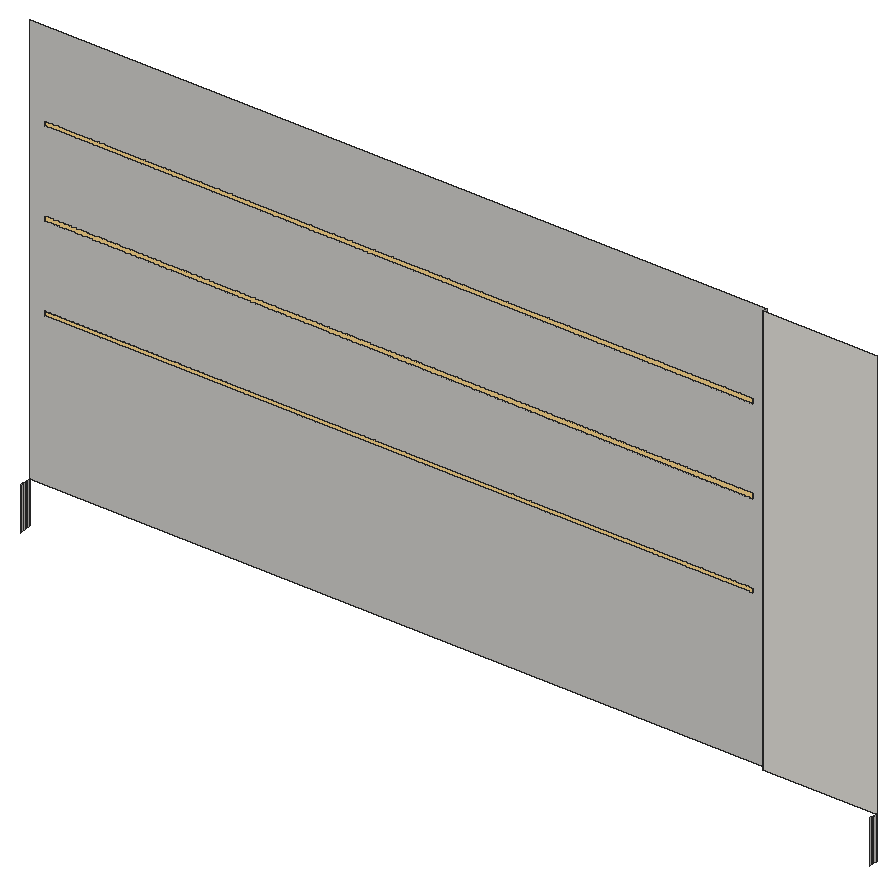
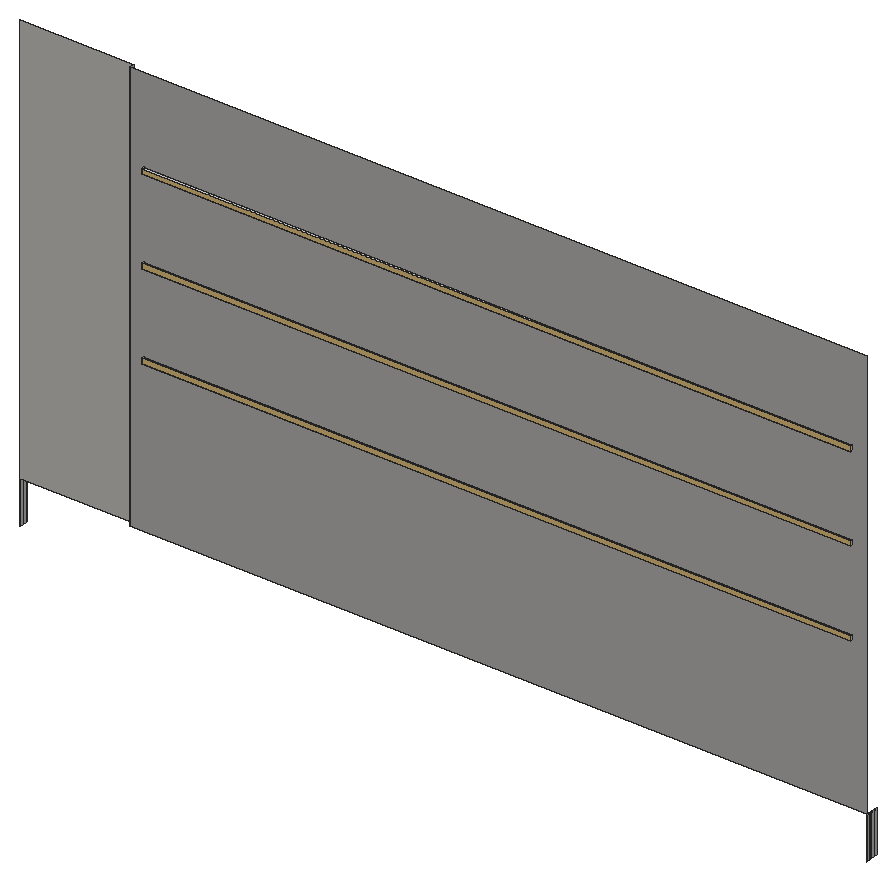
# SketchUp Ruby script. Lengths in inches.
U = 1.inch
M = Sketchup.active_model
def pt(a) = Geom::Point3d.new(a.map { |v| v * U })
def face(e, loops, mat)
  f = e.add_face(loops[0].map { |a| pt(a) })
  loops[1..].each { |l| e.add_face(l.map { |a| pt(a) }).erase! }
  f.material = f.back_material = mat if mat
  f
end
# faces: each face lists its corners as indices into pts; further lists are holes
def faces(e, pts, list, mat = nil) = list.each { |f| face(e, (f[0].is_a?(Array) ? f : [f]).map { |l| l.map { |i| pts[i] } }, mat) }
# xy, xz, yz: faces in a plane at the given z, y or x. An outline is a flat list of corners, or four numbers for a rectangle; further outlines are holes
def ring(l) = l.size == 4 ? [[l[0], l[1]], [l[2], l[1]], [l[2], l[3]], [l[0], l[3]]] : l.each_slice(2).to_a
def flat(e, list, mat, &to3) = list.each { |f| face(e, (f[0].is_a?(Array) ? f : [f]).map { |l| ring(l).map { |u, v| to3.(u, v) } }, mat) }
def xy(e, z, list, mat = nil) = flat(e, list, mat) { |x, y| [x, y, z] }
def xz(e, y, list, mat = nil) = flat(e, list, mat) { |x, z| [x, y, z] }
def yz(e, x, list, mat = nil) = flat(e, list, mat) { |y, z| [x, y, z] }
def lines(e, pts, list) = list.each { |a, b| e.add_line(pt(pts[a]), pt(pts[b])) }
# prism: a flat outline (further loops are holes) pulled along v
def prism(e, loops, v, mat = nil)
  f = face(e, loops, mat); d = Geom::Vector3d.new(v.map { |x| x * U })
  f.pushpull(f.normal.samedirection?(d) ? d.length : -d.length)
end
def box(e, o, s, mat = nil) = prism(e, [[o, [o[0] + s[0], o[1], o[2]], [o[0] + s[0], o[1] + s[1], o[2]], [o[0], o[1] + s[1], o[2]]]], [0, 0, s[2]], mat)
def at(x, y, z, deg = 0) = Geom::Transformation.translation(pt([x, y, z])) * Geom::Transformation.rotation(ORIGIN, Z_AXIS, deg.degrees)
def axes(o, x, y, z) = Geom::Transformation.new([*x, 0, *y, 0, *z, 0, *pt(o).to_a, 1])
def part(name) = M.definitions.add(name)
# library, detail: a bought-in or finely detailed component or shape, given as its bounding box
def library(name, o, s) = part(name).tap { |d| box(d.entities, o, s) }
def detail(e, o, s) = box(e.add_group.entities, o, s)
def put(e, d, t, mat = nil) = e.add_instance(d, t).tap { |i| i.material = mat if mat }
def group(e, t, mat = nil) = e.add_group.tap { |g| g.transformation = t; g.material = mat if mat }.entities
root = M.entities
M.materials.add("Outer Light - 1").color = [251, 216, 141]
M.materials.add("[Quartz Light Brown]").color = [215, 212, 212]
M.materials.add("[Stone Sandstone Ashlar Light]").color = [201, 199, 196]
M.materials.add("[Terrazzo Tile Light]").color = [219, 217, 210]
c1 = part("Group\#57")
box(c1.entities,[0,-0.5,0],[150,0.5,1])
xy(root,29,[[219,37,369,37.5]],"[Quartz Light Brown]")
xy(root,30,[[219,37,369,37.5]],"[Quartz Light Brown]")
xy(root,47,[[219,37,369,37.5]],"[Quartz Light Brown]")
xy(root,48,[[219,37,369,37.5]],"[Quartz Light Brown]")
xy(root,65,[[219,37,369,37.5]],"[Quartz Light Brown]")
xy(root,66,[[219,37,369,37.5]],"[Quartz Light Brown]")
xz(root,36,[[395.99,-12,396,-12,396,84,372,84,372,-3,395.99,-3]],"[Terrazzo Tile Light]")
xz(root,37,[[[216,-3,372,84],[219,65,369,66],[219,47,369,48],[219,29,369,30]]],"[Stone Sandstone Ashlar Light]")
xz(root,37.5,[[219,29,369,30],[219,47,369,48],[219,65,369,66]],"[Quartz Light Brown]")
yz(root,216,[[36.61,-12,37,-3]],"[Stone Sandstone Ashlar Light]")
yz(root,219,[[37,29,37.5,30],[37,47,37.5,48],[37,65,37.5,66]],"[Quartz Light Brown]")
yz(root,369,[[37,29,37.5,30],[37,47,37.5,48],[37,65,37.5,66]],"[Quartz Light Brown]")
yz(root,372,[[36,-3,37,84]],"[Stone Sandstone Ashlar Light]")
p = [[216.09,34.28,-3],[216.07,34.67,-3],[216.07,34.67,-12],[216.09,34.28,-12],[395.93,34.67,-3],[395.91,34.28,-3],
  [395.91,34.28,-12],[395.93,34.67,-12],[216.05,35.06,-3],[216.05,35.06,-12],[395.95,35.06,-3],[395.95,35.06,-12],
  [216.03,35.45,-3],[216.03,35.45,-12],[395.97,35.45,-3],[395.97,35.45,-12],[216.02,35.83,-3],[216.02,35.83,-12],
  [395.98,35.83,-3],[395.98,35.83,-12],[216.01,36.22,-3],[216.01,36.22,-12],[395.99,36,-3],[395.99,36,-12],
  [216,36.61,-3],[216,36.61,-12],[396,37,-3],[396,36.61,-3],[395.99,36.22,-3],[516.01,36,-12],
  [516,36,-12]]
faces(root,p,[[0,1,2,3],[4,5,6,7],[1,8,9,2],[10,4,7,11],[8,12,13,9],[14,10,11,15],[12,16,17,13],[18,14,15,19],
  [16,20,21,17],[22,18,19,23],[20,24,25,21]],"[Stone Sandstone Ashlar Light]")
lines(root,p,[[26,27],[27,28],[28,22],[29,30]])
put(root,c1,at(219,37.5,29),"Outer Light - 1")
put(root,c1,at(219,37.5,47),"Outer Light - 1")
put(root,c1,at(219,37.5,65),"Outer Light - 1")
